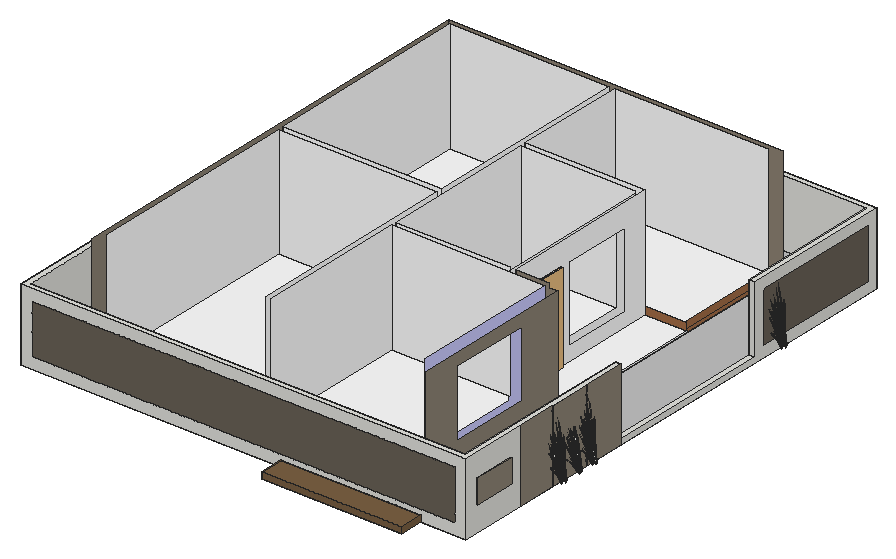
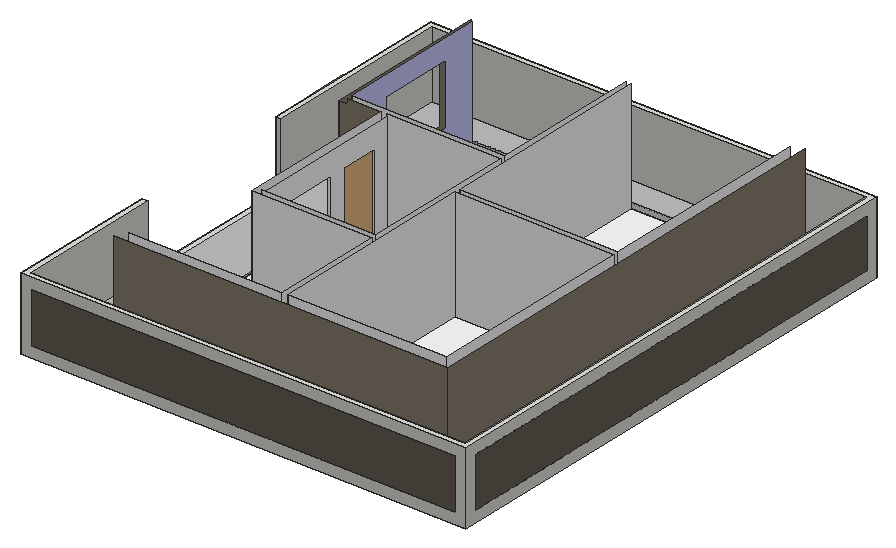
# SketchUp Ruby script. Lengths in inches.
U = 1.inch
M = Sketchup.active_model
def pt(a) = Geom::Point3d.new(a.map { |v| v * U })
def face(e, loops, mat)
  f = e.add_face(loops[0].map { |a| pt(a) })
  loops[1..].each { |l| e.add_face(l.map { |a| pt(a) }).erase! }
  f.material = f.back_material = mat if mat
  f
end
# faces: each face lists its corners as indices into pts; further lists are holes
def faces(e, pts, list, mat = nil) = list.each { |f| face(e, (f[0].is_a?(Array) ? f : [f]).map { |l| l.map { |i| pts[i] } }, mat) }
# xy, xz, yz: faces in a plane at the given z, y or x. An outline is a flat list of corners, or four numbers for a rectangle; further outlines are holes
def ring(l) = l.size == 4 ? [[l[0], l[1]], [l[2], l[1]], [l[2], l[3]], [l[0], l[3]]] : l.each_slice(2).to_a
def flat(e, list, mat, &to3) = list.each { |f| face(e, (f[0].is_a?(Array) ? f : [f]).map { |l| ring(l).map { |u, v| to3.(u, v) } }, mat) }
def xy(e, z, list, mat = nil) = flat(e, list, mat) { |x, y| [x, y, z] }
def xz(e, y, list, mat = nil) = flat(e, list, mat) { |x, z| [x, y, z] }
def yz(e, x, list, mat = nil) = flat(e, list, mat) { |y, z| [x, y, z] }
def lines(e, pts, list) = list.each { |a, b| e.add_line(pt(pts[a]), pt(pts[b])) }
# prism: a flat outline (further loops are holes) pulled along v
def prism(e, loops, v, mat = nil)
  f = face(e, loops, mat); d = Geom::Vector3d.new(v.map { |x| x * U })
  f.pushpull(f.normal.samedirection?(d) ? d.length : -d.length)
end
def box(e, o, s, mat = nil) = prism(e, [[o, [o[0] + s[0], o[1], o[2]], [o[0] + s[0], o[1] + s[1], o[2]], [o[0], o[1] + s[1], o[2]]]], [0, 0, s[2]], mat)
def at(x, y, z, deg = 0) = Geom::Transformation.translation(pt([x, y, z])) * Geom::Transformation.rotation(ORIGIN, Z_AXIS, deg.degrees)
def axes(o, x, y, z) = Geom::Transformation.new([*x, 0, *y, 0, *z, 0, *pt(o).to_a, 1])
def part(name) = M.definitions.add(name)
# library, detail: a bought-in or finely detailed component or shape, given as its bounding box
def library(name, o, s) = part(name).tap { |d| box(d.entities, o, s) }
def detail(e, o, s) = box(e.add_group.entities, o, s)
def put(e, d, t, mat = nil) = e.add_instance(d, t).tap { |i| i.material = mat if mat }
def group(e, t, mat = nil) = e.add_group.tap { |g| g.transformation = t; g.material = mat if mat }.entities
root = M.entities
M.materials.add("I01_Sky_Frost").color = [204, 204, 255]
M.materials.add("LightPink_Translucent").color = [144, 107, 117]
M.materials["LightPink_Translucent"].alpha = 0.75
M.materials.add("M00_Soft_Cloud").color = [255, 255, 255]
M.materials.add("M07_Charcoal_Gleam").color = [58, 58, 58]
M.materials.add("Plaster_04_1K").color = [142, 132, 117]
M.materials.add("Plaster_04_1K1").color = [106, 98, 87]
M.materials.add("Soil_03_1K").color = [122, 96, 67]
M.materials.add("Wood_Veneer_15_1K").color = [163, 109, 71]
M.materials.add("[Metal_Corrogated_Shiny]").color = [193, 193, 193]
c1 = library("porta+4",[0.2,-5.42,1.33],[46.55,4.72,83.21])
c2 = part("blade")
p = [[2.15,0.21,22],[0,0.17,0],[0.09,0.45,0],[2.18,0.31,22],[2.29,0.31,22],[0.38,0.45,0],
  [2.48,0.24,33],[2.49,0.24,33],[2.48,0.22,33]]
faces(c2.entities,p,[[0,1,2,3],[4,5,2,3],[6,3,4,7],[8,0,3,6]])
c3 = part("seeds")
p = [[0.3,-0.1,1.38],[-0.01,-0.03,1.59],[-0.01,-0.03,0.03],[0.14,-0.07,-0.07],[0.29,-0.03,3],[0.15,0.01,3.11]]
faces(c3.entities,p,[[0,1,2,3],[1,0,4,5]],"LightPink_Translucent")
c4 = part("blade with seeds")
put(c4.entities,c2,at(0,0,0))
put(c4.entities,c3,axes([2.4,0.25,30.99],[1.5799,-0.05474,1.17369],[-0.12525,1.92788,0.29478],[-0.07173,-0.02425,1.56792]))
xy(root,-6,[[280.62,2.62,431.17,27.98],[[0,27.98,480,579.98],[48.29,63.98,409.55,544.6]]])
xy(root,-6,[[48,63.98,408,543.98]],"M00_Soft_Cloud")
xy(root,0,[[474,236.51,480,416.03]])
xy(root,0,[[57,72.98,228,303.98],[234,72.98,399,234.98],[234,240.98,357,408.98],[363,240.98,408,414.98],[57,309.98,228,534.98],
  [234,414.98,399,534.98]],"M00_Soft_Cloud")
xy(root,0,[[[6,33.98,474,573.98],[48.29,63.98,409.55,544.6]]],"[Metal_Corrogated_Shiny]")
xy(root,0.58,[[280.62,2.62,431.17,27.98]],"Soil_03_1K")
xy(root,3,[[357,255.98,363,297.98]],"M00_Soft_Cloud")
xy(root,22.44,[[480,40.97,482,86.92]],"Plaster_04_1K")
xy(root,48.1875,[[480,40.97,482,86.92]],"Plaster_04_1K")
xy(root,72,[[0,27.98,480,27.98,480,236.51,474,236.51,474,33.98,6,33.98,6,573.98,474,573.98,474,416.03,480,416.03,480,579.98,0,579.98]])
xz(root,2.62,[[280.62,-6,431.17,0.58]],"Soil_03_1K")
xz(root,27.98,[[[0,-6,280.62,-6,280.62,0.58,431.17,0.58,431.17,-6,480,-6,480,72,0,72],[12,6,468,60]],[280.62,-6,431.17,0.58]])
xz(root,27.98,[[12,6,468,60]],"Plaster_04_1K1")
xz(root,33.98,[[6,0,474,72]])
xz(root,40.97,[[480,22.44,482,48.1875]],"Plaster_04_1K")
xz(root,63.98,[[48,-6,48.29,0],[48.29,-6,409.55,0]])
xz(root,86.92,[[480,22.44,482,48.1875]],"Plaster_04_1K")
xz(root,234.98,[[234,0,399,120]],"M00_Soft_Cloud")
xz(root,236.51,[[474,0,480,72]])
xz(root,240.98,[[234,0,357,120]],"M00_Soft_Cloud")
xz(root,240.98,[[363,0,363,120,399,120,399,114.97,408,114.97,408,0]],"Plaster_04_1K")
xz(root,255.98,[[357,3,363,93]],"M00_Soft_Cloud")
xz(root,297.98,[[357,3,363,93]],"M00_Soft_Cloud")
xz(root,303.98,[[57,0,228,120]],"M00_Soft_Cloud")
xz(root,309.98,[[57,0,228,120]],"M00_Soft_Cloud")
xz(root,408.98,[[234,0,357,120]],"M00_Soft_Cloud")
xz(root,414.98,[[234,0,363,120]],"M00_Soft_Cloud")
xz(root,414.98,[[363,0,408,8.21]],"Wood_Veneer_15_1K")
xz(root,416.03,[[474,0,480,72]])
xz(root,534.98,[[57,0,228,120],[234,0,399,120]],"M00_Soft_Cloud")
xz(root,543.98,[[48,-6,408,117]],"Plaster_04_1K")
xz(root,544.6,[[48.29,-6,409.55,0]])
xz(root,573.98,[[6,0,474,72]])
xz(root,579.98,[[[0,-6,480,72],[12,6,468,60]]])
xz(root,579.98,[[12,6,468,60]],"Plaster_04_1K1")
yz(root,0,[[[27.98,-6,579.98,72],[39.98,6,567.98,60]]])
yz(root,0,[[39.98,6,567.98,60]],"Plaster_04_1K1")
yz(root,6,[[33.98,0,573.98,72]])
yz(root,48,[[63.98,-6,543.98,117]],"Plaster_04_1K")
yz(root,48.29,[[63.98,-6,544.6,0]])
yz(root,57,[[72.98,0,303.98,120],[309.98,0,534.98,120]],"M00_Soft_Cloud")
yz(root,228,[[72.98,0,303.98,120],[309.98,0,534.98,120]],"M00_Soft_Cloud")
yz(root,234,[[72.98,0,234.98,120],[240.98,0,408.98,120],[414.98,0,534.98,120]],"M00_Soft_Cloud")
yz(root,280.62,[[2.62,-6,27.98,0.58]],"Soil_03_1K")
yz(root,357,[[[240.98,0,408.98,117],[315.98,18,384.98,93],[255.98,3,297.98,93]]],"M00_Soft_Cloud")
yz(root,363,[[[240.98,0,252.98,0,252.98,96,300.98,96,300.98,0,414.98,0,414.98,120,240.98,120],[312.98,15,387.98,96]],[[252.98,0,300.98,96],[255.98,3,297.98,93]]],"M00_Soft_Cloud")
yz(root,399,[[[72.98,0,234.98,120],[111.98,30,186.98,30,186.98,33,189.98,33,189.98,99,108.98,99,108.98,33,111.98,33]]],"I01_Sky_Frost")
yz(root,408,[[240.98,-6,414.98,0]],"M00_Soft_Cloud")
yz(root,408,[[[63.98,-6,240.98,114.97],[105.98,30,192.98,102]]],"Plaster_04_1K")
yz(root,408,[[414.98,-6,543.98,2.03],[414.98,2.03,543.98,10.05]],"Wood_Veneer_15_1K")
yz(root,409.55,[[63.98,-6,544.6,0]])
yz(root,431.17,[[2.62,-6,27.98,0.58]],"Soil_03_1K")
yz(root,474,[[33.98,0,236.51,72],[416.03,0,573.98,72]])
yz(root,480,[[[27.98,-6,99.98,72],[40.97,22.44,86.92,48.1875]],[[236.51,-6,579.98,-6,579.98,72,416.03,72,416.03,0,236.51,0],[428.03,6,567.98,60]]])
yz(root,480,[[143.49,-6,145.49,72],[189,-6,191,72]],"M07_Charcoal_Gleam")
yz(root,480,[[99.98,-6,143.49,72],[145.49,-6,189,72],[191,-6,236.51,72]],"Plaster_04_1K")
yz(root,480,[[428.03,6,567.98,60]],"Plaster_04_1K1")
yz(root,482,[[40.97,22.44,86.92,48.1875]],"Plaster_04_1K")
p = [[363,408.98,0],[357,408.98,0]]
lines(root,p,[[0,1]])
put(root,c1,axes([360.24,254.23,-1.54],[0,1,0],[-1,0,0],[0,0,1.15408]))
put(root,c4,axes([489.51,442.16,3.07],[0.31515,-0.01384,1.71376],[-0.20907,0.5998,0.13857],[-0.44912,-0.0371,0.73262]))
put(root,c4,axes([489.58,145.76,3.07],[0.31515,-0.01384,1.71376],[-0.20907,0.5998,0.13857],[-0.44912,-0.0371,0.73262]))
put(root,c4,axes([489.65,186.83,3.07],[0.31515,-0.01384,1.71376],[-0.20907,0.5998,0.13857],[-0.44912,-0.0371,0.73262]))
put(root,c4,axes([489.64,443.21,3.07],[0.26363,-0.12925,1.71376],[0.22195,0.59723,0.13857],[-0.41388,0.13498,0.73262]))
put(root,c4,axes([489.71,146.8125,3.07],[0.26363,-0.12925,1.71376],[0.22195,0.59723,0.13857],[-0.41388,0.13498,0.73262]))
put(root,c4,axes([489.78,187.88,3.07],[0.26363,-0.12925,1.71376],[0.22195,0.59723,0.13857],[-0.41388,0.13498,0.73262]))
put(root,c4,axes([488.82,444.23,1.78],[0.26405,0.05016,1.43002],[0.17019,0.51235,-0.30754],[-0.35868,0.0959,0.61141]))
put(root,c4,axes([488.89,147.83,1.78],[0.26405,0.05016,1.43002],[0.17019,0.51235,-0.30754],[-0.35868,0.0959,0.61141]))
put(root,c4,axes([488.96,188.9,1.78],[0.26405,0.05016,1.43002],[0.17019,0.51235,-0.30754],[-0.35868,0.0959,0.61141]))
put(root,c4,axes([491.15,442.59,2.53],[0.21597,-0.08839,1.77064],[0.07448,0.61717,0.13857],[-0.4678,0.08189,0.63284]))
put(root,c4,axes([491.23,146.1875,2.53],[0.21597,-0.08839,1.77064],[0.07448,0.61717,0.13857],[-0.4678,0.08189,0.63284]))
put(root,c4,axes([491.3,187.26,2.53],[0.21597,-0.08839,1.77064],[0.07448,0.61717,0.13857],[-0.4678,0.08189,0.63284]))
put(root,c4,axes([491.2,165.89,3.07],[0.31515,-0.01384,1.71376],[-0.20907,0.5998,0.13857],[-0.44912,-0.0371,0.73262]))
put(root,c4,axes([488.83,443,3.91],[-0.12407,0.07933,1.74944],[0.01055,0.57963,-0.27667],[-0.2844,0.07538,0.14031]))
put(root,c4,axes([490.45,441.6,4.17],[-0.75952,-0.01471,-0.71045],[0.05101,-0.61953,0.08574],[-0.32177,-0.06538,1.00501]))
put(root,c4,axes([488.91,146.6,3.91],[-0.12407,0.07933,1.74944],[0.01055,0.57963,-0.27667],[-0.2844,0.07538,0.14031]))
put(root,c4,axes([490.53,145.2,4.17],[-0.75952,-0.01471,-0.71045],[0.05101,-0.61953,0.08574],[-0.32177,-0.06538,1.00501]))
put(root,c4,axes([489.84,441.75,1.78],[0.14835,0.17012,1.43002],[-0.34183,0.46242,-0.30754],[-0.351,-0.11053,0.61141]))
put(root,c4,axes([488.98,187.67,3.91],[-0.12407,0.07933,1.74944],[0.01055,0.57963,-0.27667],[-0.2844,0.07538,0.14031]))
put(root,c4,axes([490.59,186.27,4.17],[-0.75952,-0.01471,-0.71045],[0.05101,-0.61953,0.08574],[-0.32177,-0.06538,1.00501]))
put(root,c4,axes([489.91,145.35,1.78],[0.14835,0.17012,1.43002],[-0.34183,0.46242,-0.30754],[-0.351,-0.11053,0.61141]))
put(root,c4,axes([489.23,442.67,3.72],[-0.63144,-0.17046,-0.35414],[0.18417,-0.49731,0.4572],[-0.25423,0.0456,0.87481]))
put(root,c4,axes([489.98,186.42,1.78],[0.14835,0.17012,1.43002],[-0.34183,0.46242,-0.30754],[-0.351,-0.11053,0.61141]))
put(root,c4,axes([490.1,441.19,3.07],[0.28223,0.10528,1.71376],[-0.58406,0.44165,0.13857],[-0.36402,-0.19924,0.73262]))
put(root,c4,axes([489.3,146.27,3.72],[-0.63144,-0.17046,-0.35414],[0.18417,-0.49731,0.4572],[-0.25423,0.0456,0.87481]))
put(root,c4,axes([490.18,144.79,3.07],[0.28223,0.10528,1.71376],[-0.58406,0.44165,0.13857],[-0.36402,-0.19924,0.73262]))
put(root,c4,axes([489.375,187.34,3.72],[-0.63144,-0.17046,-0.35414],[0.18417,-0.49731,0.4572],[-0.25423,0.0456,0.87481]))
put(root,c4,axes([490.25,185.86,3.07],[0.28223,0.10528,1.71376],[-0.58406,0.44165,0.13857],[-0.36402,-0.19924,0.73262]))
put(root,c4,axes([487.45,443.59,3.9],[0.09697,0.01639,1.77383],[0.29997,0.53988,-0.16761],[-0.1985,0.1417,0.31391]))
put(root,c4,axes([489.66,442.92,3.875],[-0.20584,0.55581,-0.51099],[-0.70573,-0.19051,-0.3958],[-0.28414,0.05097,0.97773]))
put(root,c4,axes([487.53,147.1875,3.9],[0.09697,0.01639,1.77383],[0.29997,0.53988,-0.16761],[-0.1985,0.1417,0.31391]))
put(root,c4,axes([489.74,146.53,3.875],[-0.20584,0.55581,-0.51099],[-0.70573,-0.19051,-0.3958],[-0.28414,0.05097,0.97773]))
put(root,c4,axes([487.6,188.26,3.9],[0.09697,0.01639,1.77383],[0.29997,0.53988,-0.16761],[-0.1985,0.1417,0.31391]))
put(root,c4,axes([489.81,187.59,3.875],[-0.20584,0.55581,-0.51099],[-0.70573,-0.19051,-0.3958],[-0.28414,0.05097,0.97773]))
put(root,c4,axes([490.2,441.72,3.875],[-0.55171,0.40476,-0.51099],[-0.48318,-0.42758,-0.3958],[-0.28031,-0.06159,0.97773]))
put(root,c4,axes([489.31,442.89,0.6875],[0.01927,0.0963,1.76342],[-0.38846,0.5029,-0.26939],[-0.27592,-0.02535,0.30037]))
put(root,c4,axes([491.33,166.95,3.07],[0.26363,-0.12925,1.71376],[0.22195,0.59723,0.13857],[-0.41388,0.13498,0.73262]))
put(root,c4,axes([490.27,145.32,3.875],[-0.55171,0.40476,-0.51099],[-0.48318,-0.42758,-0.3958],[-0.28031,-0.06159,0.97773]))
put(root,c4,axes([489.38,146.49,0.6875],[0.01927,0.0963,1.76342],[-0.38846,0.5029,-0.26939],[-0.27592,-0.02535,0.30037]))
put(root,c4,axes([490.34,186.39,3.875],[-0.55171,0.40476,-0.51099],[-0.48318,-0.42758,-0.3958],[-0.28031,-0.06159,0.97773]))
put(root,c4,axes([489.45,187.56,0.6875],[0.01927,0.0963,1.76342],[-0.38846,0.5029,-0.26939],[-0.27592,-0.02535,0.30037]))
put(root,c4,axes([490.51,167.97,1.78],[0.26405,0.05016,1.43002],[0.17019,0.51235,-0.30754],[-0.35868,0.0959,0.61141]))
put(root,c4,axes([489.42,440.59,3.9],[0.05633,0.06098,1.77383],[-0.27155,0.54815,-0.16761],[-0.27501,0.00397,0.31391]))
put(root,c4,axes([489.49,144.19,3.9],[0.05633,0.06098,1.77383],[-0.27155,0.54815,-0.16761],[-0.27501,0.00397,0.31391]))
put(root,c4,axes([488.26,445.3,1.96],[0.31665,-0.27694,1.1486],[0.12495,0.43841,0.84392],[-0.22883,0.0785,0.25299]))
put(root,c4,axes([489.5625,185.26,3.9],[0.05633,0.06098,1.77383],[-0.27155,0.54815,-0.16761],[-0.27501,0.00397,0.31391]))
put(root,c4,axes([490.05,440.22,3.91],[-0.16348,-0.00431,1.74944],[-0.52047,0.43131,-0.27667],[-0.2777,-0.08813,0.14031]))
put(root,c4,axes([488.34,148.9,1.96],[0.31665,-0.27694,1.1486],[0.12495,0.43841,0.84392],[-0.22883,0.0785,0.25299]))
put(root,c4,axes([492.85,166.33,2.53],[0.21597,-0.08839,1.77064],[0.07448,0.61717,0.13857],[-0.4678,0.08189,0.63284]))
put(root,c4,axes([488.41,189.97,1.96],[0.31665,-0.27694,1.1486],[0.12495,0.43841,0.84392],[-0.22883,0.0785,0.25299]))
put(root,c4,axes([490.12,143.82,3.91],[-0.16348,-0.00431,1.74944],[-0.52047,0.43131,-0.27667],[-0.2777,-0.08813,0.14031]))
put(root,c4,axes([489.375,442.61,3.93],[0.21466,-0.55714,0.48003],[0.70573,0.19051,0.3958],[-0.27753,0.03348,0.9933]))
put(root,c4,axes([490.19,184.89,3.91],[-0.16348,-0.00431,1.74944],[-0.52047,0.43131,-0.27667],[-0.2777,-0.08813,0.14031]))
put(root,c4,axes([489.625,442.45,4.23],[0.38229,0.5533,-0.1216],[-0.6785,0.2719,-0.67495],[-0.28593,0.073,1.02557]))
put(root,c4,axes([489.45,146.21,3.93],[0.21466,-0.55714,0.48003],[0.70573,0.19051,0.3958],[-0.27753,0.03348,0.9933]))
put(root,c4,axes([490.49,441.3,4.23],[-0.04068,0.62141,-0.1216],[-0.77029,-0.01698,-0.67495],[-0.29667,-0.04317,1.02557]))
put(root,c4,axes([489.99,441.34,3.72],[-0.43232,-0.38257,-0.35414],[0.49364,-0.36215,0.4572],[-0.25081,-0.0551,0.87481]))
put(root,c4,axes([489.7,146.05,4.23],[0.38229,0.5533,-0.1216],[-0.6785,0.2719,-0.67495],[-0.28593,0.073,1.02557]))
put(root,c4,axes([489.52,187.28,3.93],[0.21466,-0.55714,0.48003],[0.70573,0.19051,0.3958],[-0.27753,0.03348,0.9933]))
put(root,c4,axes([489.32,442.46,3.92],[-0.27906,-0.41663,0.0643],[0.50888,-0.20393,0.50621],[-0.22432,0.04024,0.77189]))
put(root,c4,axes([490.5625,144.9,4.23],[-0.04068,0.62141,-0.1216],[-0.77029,-0.01698,-0.67495],[-0.29667,-0.04317,1.02557]))
put(root,c4,axes([490.07,144.94,3.72],[-0.43232,-0.38257,-0.35414],[0.49364,-0.36215,0.4572],[-0.25081,-0.0551,0.87481]))
put(root,c4,axes([489.77,187.12,4.23],[0.38229,0.5533,-0.1216],[-0.6785,0.2719,-0.67495],[-0.28593,0.073,1.02557]))
put(root,c4,axes([490.6,443.61,3.07],[0.18977,-0.18775,1.71376],[0.47917,0.50677,0.13857],[-0.32866,0.23079,0.73262]))
put(root,c4,axes([489.46,444.11,3.72],[-0.66138,0.08733,-0.35414],[-0.17464,-0.49921,0.4572],[-0.18953,0.13408,0.87481]))
put(root,c4,axes([489.4,146.0625,3.92],[-0.27906,-0.41663,0.0643],[0.50888,-0.20393,0.50621],[-0.22432,0.04024,0.77189]))
put(root,c4,axes([490.63,185.97,4.23],[-0.04068,0.62141,-0.1216],[-0.77029,-0.01698,-0.67495],[-0.29667,-0.04317,1.02557]))
put(root,c4,axes([490.14,186.01,3.72],[-0.43232,-0.38257,-0.35414],[0.49364,-0.36215,0.4572],[-0.25081,-0.0551,0.87481]))
put(root,c4,axes([490.68,147.21,3.07],[0.18977,-0.18775,1.71376],[0.47917,0.50677,0.13857],[-0.32866,0.23079,0.73262]))
put(root,c4,axes([489.47,187.13,3.92],[-0.27906,-0.41663,0.0643],[0.50888,-0.20393,0.50621],[-0.22432,0.04024,0.77189]))
put(root,c4,axes([489.54,147.71,3.72],[-0.66138,0.08733,-0.35414],[-0.17464,-0.49921,0.4572],[-0.18953,0.13408,0.87481]))
put(root,c4,axes([490.75,188.28,3.07],[0.18977,-0.18775,1.71376],[0.47917,0.50677,0.13857],[-0.32866,0.23079,0.73262]))
put(root,c4,axes([489.61,188.78,3.72],[-0.66138,0.08733,-0.35414],[-0.17464,-0.49921,0.4572],[-0.18953,0.13408,0.87481]))
put(root,c4,axes([489.1,445.59,0.6875],[0.10192,0.06105,1.76342],[0.17281,0.56562,-0.26939],[-0.22588,0.12062,0.30037]))
put(root,c4,axes([490.53,166.74,3.91],[-0.12407,0.07933,1.74944],[0.01055,0.57963,-0.27667],[-0.2844,0.07538,0.14031]))
put(root,c4,axes([492.14,165.34,4.17],[-0.75952,-0.01471,-0.71045],[0.05101,-0.61953,0.08574],[-0.32177,-0.06538,1.00501]))
put(root,c4,axes([488.95,442.26,1.96],[0.48508,-0.04372,1.1486],[-0.3077,0.38525,0.84392],[-0.23971,-0.05779,0.25299]))
put(root,c4,axes([489.18,149.1875,0.6875],[0.10192,0.06105,1.76342],[0.17281,0.56562,-0.26939],[-0.22588,0.12062,0.30037]))
put(root,c4,axes([491.53,165.49,1.78],[0.14835,0.17012,1.43002],[-0.34183,0.46242,-0.30754],[-0.351,-0.11053,0.61141]))
put(root,c4,axes([489.03,145.86,1.96],[0.48508,-0.04372,1.1486],[-0.3077,0.38525,0.84392],[-0.23971,-0.05779,0.25299]))
put(root,c4,axes([489.24,190.26,0.6875],[0.10192,0.06105,1.76342],[0.17281,0.56562,-0.26939],[-0.22588,0.12062,0.30037]))
put(root,c4,axes([489.1,186.93,1.96],[0.48508,-0.04372,1.1486],[-0.3077,0.38525,0.84392],[-0.23971,-0.05779,0.25299]))
put(root,c4,axes([490.92,166.41,3.72],[-0.63144,-0.17046,-0.35414],[0.18417,-0.49731,0.4572],[-0.25423,0.0456,0.87481]))
put(root,c4,axes([489.54,444,3.93],[-0.18844,-0.56237,0.48003],[0.73919,-0.0976,0.3958],[-0.21785,0.13226,0.9933]))
put(root,c4,axes([491.8,164.93,3.07],[0.28223,0.10528,1.71376],[-0.58406,0.44165,0.13857],[-0.36402,-0.19924,0.73262]))
put(root,c4,axes([489.62,147.6,3.93],[-0.18844,-0.56237,0.48003],[0.73919,-0.0976,0.3958],[-0.21785,0.13226,0.9933]))
put(root,c4,axes([489.93,441.2,4.29],[0.62747,-0.45094,0.53763],[0.54116,0.47889,0.4433],[-0.29439,-0.08318,1.11249]))
put(root,c4,axes([489.69,188.67,3.93],[-0.18844,-0.56237,0.48003],[0.73919,-0.0976,0.3958],[-0.21785,0.13226,0.9933]))
put(root,c4,axes([489.4,443.89,3.92],[-0.52161,-0.25698,0.0643],[0.30368,-0.36595,0.50621],[-0.16723,0.11831,0.77189]))
put(root,c4,axes([490,144.8,4.29],[0.62747,-0.45094,0.53763],[0.54116,0.47889,0.4433],[-0.29439,-0.08318,1.11249]))
put(root,c4,axes([489.15,167.33,3.9],[0.09697,0.01639,1.77383],[0.29997,0.53988,-0.16761],[-0.1985,0.1417,0.31391]))
put(root,c4,axes([489.48,147.49,3.92],[-0.52161,-0.25698,0.0643],[0.30368,-0.36595,0.50621],[-0.16723,0.11831,0.77189]))
put(root,c4,axes([490.07,185.87,4.29],[0.62747,-0.45094,0.53763],[0.54116,0.47889,0.4433],[-0.29439,-0.08318,1.11249]))
put(root,c4,axes([491.36,166.66,3.875],[-0.20584,0.55581,-0.51099],[-0.70573,-0.19051,-0.3958],[-0.28414,0.05097,0.97773]))
put(root,c4,axes([489.55,188.56,3.92],[-0.52161,-0.25698,0.0643],[0.30368,-0.36595,0.50621],[-0.16723,0.11831,0.77189]))
put(root,c4,axes([491.89,165.46,3.875],[-0.55171,0.40476,-0.51099],[-0.48318,-0.42758,-0.3958],[-0.28031,-0.06159,0.97773]))
put(root,c4,axes([490.46,444.08,3.07],[0.14147,-0.21002,1.71376],[0.59349,0.43464,0.13857],[-0.26773,0.27089,0.73262]))
put(root,c4,axes([491,166.63,0.6875],[0.01927,0.0963,1.76342],[-0.38846,0.5029,-0.26939],[-0.27592,-0.02535,0.30037]))
put(root,c4,axes([490.54,147.68,3.07],[0.14147,-0.21002,1.71376],[0.59349,0.43464,0.13857],[-0.26773,0.27089,0.73262]))
put(root,c4,axes([490.61,188.75,3.07],[0.14147,-0.21002,1.71376],[0.59349,0.43464,0.13857],[-0.26773,0.27089,0.73262]))
put(root,c4,axes([491.11,164.33,3.9],[0.05633,0.06098,1.77383],[-0.27155,0.54815,-0.16761],[-0.27501,0.00397,0.31391]))
put(root,c4,axes([489.89,442.62,4.24],[0.63144,0.17046,0.35414],[-0.18417,0.49731,-0.4572],[-0.25423,0.0456,0.87481]))
put(root,c4,axes([489.97,146.22,4.24],[0.63144,0.17046,0.35414],[-0.18417,0.49731,-0.4572],[-0.25423,0.0456,0.87481]))
put(root,c4,axes([490,444.16,3.875],[0.19519,0.55794,-0.51099],[-0.73919,0.0976,-0.3958],[-0.21183,0.14986,0.97773]))
put(root,c4,axes([489.96,169.04,1.96],[0.31665,-0.27694,1.1486],[0.12495,0.43841,0.84392],[-0.22883,0.0785,0.25299]))
put(root,c4,axes([490.04,187.29,4.24],[0.63144,0.17046,0.35414],[-0.18417,0.49731,-0.4572],[-0.25423,0.0456,0.87481]))
put(root,c4,axes([491.74,163.96,3.91],[-0.16348,-0.00431,1.74944],[-0.52047,0.43131,-0.27667],[-0.2777,-0.08813,0.14031]))
put(root,c4,axes([490.08,147.76,3.875],[0.19519,0.55794,-0.51099],[-0.73919,0.0976,-0.3958],[-0.21183,0.14986,0.97773]))
put(root,c4,axes([490.21,441.2,3.92],[0.03826,-0.46465,0.0643],[0.57772,0.01274,0.50621],[-0.2213,-0.04862,0.77189]))
put(root,c4,axes([488.85,445.17,3.91],[-0.01889,0.12092,1.74944],[0.53598,0.42065,-0.27667],[-0.14032,0.19892,0.14031]))
put(root,c4,axes([490.15,188.83,3.875],[0.19519,0.55794,-0.51099],[-0.73919,0.0976,-0.3958],[-0.21183,0.14986,0.97773]))
put(root,c4,axes([490.29,144.8,3.92],[0.03826,-0.46465,0.0643],[0.57772,0.01274,0.50621],[-0.2213,-0.04862,0.77189]))
put(root,c4,axes([488.93,148.77,3.91],[-0.01889,0.12092,1.74944],[0.53598,0.42065,-0.27667],[-0.14032,0.19892,0.14031]))
put(root,c4,axes([491.85,443.76,1.25],[-0.79037,-0.10018,-0.62353],[0.16679,-0.61794,-0.16365],[-0.23587,-0.07488,1.37633]))
put(root,c4,axes([491.99,440.39,4.62],[-0.50709,0.58578,-0.13619],[-0.73436,-0.33748,-0.75594],[-0.25527,-0.1655,1.14864]))
put(root,c4,axes([491.07,166.35,3.93],[0.21466,-0.55714,0.48003],[0.70573,0.19051,0.3958],[-0.27753,0.03348,0.9933]))
put(root,c4,axes([490.36,185.87,3.92],[0.03826,-0.46465,0.0643],[0.57772,0.01274,0.50621],[-0.2213,-0.04862,0.77189]))
put(root,c4,axes([489,189.84,3.91],[-0.01889,0.12092,1.74944],[0.53598,0.42065,-0.27667],[-0.14032,0.19892,0.14031]))
put(root,c4,axes([491.92,147.36,1.25],[-0.79037,-0.10018,-0.62353],[0.16679,-0.61794,-0.16365],[-0.23587,-0.07488,1.37633]))
put(root,c4,axes([491.32,166.1875,4.23],[0.38229,0.5533,-0.1216],[-0.6785,0.2719,-0.67495],[-0.28593,0.073,1.02557]))
put(root,c4,axes([492.07,143.99,4.62],[-0.50709,0.58578,-0.13619],[-0.73436,-0.33748,-0.75594],[-0.25527,-0.1655,1.14864]))
put(root,c4,axes([490.6,441.54,4.24],[0.43232,0.38257,0.35414],[-0.49364,0.36215,-0.4572],[-0.25081,-0.0551,0.87481]))
put(root,c4,axes([492.18,165.04,4.23],[-0.04068,0.62141,-0.1216],[-0.77029,-0.01698,-0.67495],[-0.29667,-0.04317,1.02557]))
put(root,c4,axes([491.99,188.43,1.25],[-0.79037,-0.10018,-0.62353],[0.16679,-0.61794,-0.16365],[-0.23587,-0.07488,1.37633]))
put(root,c4,axes([491.6875,165.08,3.72],[-0.43232,-0.38257,-0.35414],[0.49364,-0.36215,0.4572],[-0.25081,-0.0551,0.87481]))
put(root,c4,axes([492.14,185.0625,4.62],[-0.50709,0.58578,-0.13619],[-0.73436,-0.33748,-0.75594],[-0.25527,-0.1655,1.14864]))
put(root,c4,axes([491.02,166.2,3.92],[-0.27906,-0.41663,0.0643],[0.50888,-0.20393,0.50621],[-0.22432,0.04024,0.77189]))
put(root,c4,axes([490.68,145.14,4.24],[0.43232,0.38257,0.35414],[-0.49364,0.36215,-0.4572],[-0.25081,-0.0551,0.87481]))
put(root,c4,axes([491.77,440.87,4.17],[-0.64788,-0.29534,-0.71045],[0.46044,-0.51755,0.08574],[-0.23473,-0.17635,1.00501]))
put(root,c4,axes([491.47,440.88,3.875],[-0.74975,0.14525,-0.51099],[-0.13115,-0.55007,-0.3958],[-0.20138,-0.15763,0.97773]))
put(root,c4,axes([492.3,167.35,3.07],[0.18977,-0.18775,1.71376],[0.47917,0.50677,0.13857],[-0.32866,0.23079,0.73262]))
put(root,c4,axes([490.75,186.21,4.24],[0.43232,0.38257,0.35414],[-0.49364,0.36215,-0.4572],[-0.25081,-0.0551,0.87481]))
put(root,c4,axes([491.16,167.84,3.72],[-0.66138,0.08733,-0.35414],[-0.17464,-0.49921,0.4572],[-0.18953,0.13408,0.87481]))
put(root,c4,axes([491.85,144.47,4.17],[-0.64788,-0.29534,-0.71045],[0.46044,-0.51755,0.08574],[-0.23473,-0.17635,1.00501]))
put(root,c4,axes([491.54,144.48,3.875],[-0.74975,0.14525,-0.51099],[-0.13115,-0.55007,-0.3958],[-0.20138,-0.15763,0.97773]))
put(root,c4,axes([491.91,185.54,4.17],[-0.64788,-0.29534,-0.71045],[0.46044,-0.51755,0.08574],[-0.23473,-0.17635,1.00501]))
put(root,c4,axes([491.61,185.55,3.875],[-0.74975,0.14525,-0.51099],[-0.13115,-0.55007,-0.3958],[-0.20138,-0.15763,0.97773]))
put(root,c4,axes([490.8,169.33,0.6875],[0.10192,0.06105,1.76342],[0.17281,0.56562,-0.26939],[-0.22588,0.12062,0.30037]))
put(root,c4,axes([490.81,444.93,1.21],[-0.7111,-0.30552,-0.49651],[0.42504,-0.54784,0],[-0.16196,-0.06958,1.57504]))
put(root,c4,axes([490.65,166,1.96],[0.48508,-0.04372,1.1486],[-0.3077,0.38525,0.84392],[-0.23971,-0.05779,0.25299]))
put(root,c4,axes([490.5,440.38,0.6875],[-0.0736,0.08049,1.76342],[-0.74378,0.17355,-0.26939],[-0.17968,-0.15788,0.30037]))
put(root,c4,axes([489.66,443.76,4.23],[0.70283,0.33692,-0.1216],[-0.40491,0.48793,-0.67495],[-0.19857,0.16961,1.02557]))
put(root,c4,axes([490.89,148.53,1.21],[-0.7111,-0.30552,-0.49651],[0.42504,-0.54784,0],[-0.16196,-0.06958,1.57504]))
put(root,c4,axes([490.58,143.98,0.6875],[-0.0736,0.08049,1.76342],[-0.74378,0.17355,-0.26939],[-0.17968,-0.15788,0.30037]))
put(root,c4,axes([489.73,147.36,4.23],[0.70283,0.33692,-0.1216],[-0.40491,0.48793,-0.67495],[-0.19857,0.16961,1.02557]))
put(root,c4,axes([490.96,189.6,1.21],[-0.7111,-0.30552,-0.49651],[0.42504,-0.54784,0],[-0.16196,-0.06958,1.57504]))
put(root,c4,axes([491.24,445.3,1.57],[-0.47504,0.61229,0],[-0.79476,-0.34146,-0.51607],[-0.18101,-0.07777,1.63711]))
put(root,c4,axes([490.64,185.05,0.6875],[-0.0736,0.08049,1.76342],[-0.74378,0.17355,-0.26939],[-0.17968,-0.15788,0.30037]))
put(root,c4,axes([489.8,188.43,4.23],[0.70283,0.33692,-0.1216],[-0.40491,0.48793,-0.67495],[-0.19857,0.16961,1.02557]))
put(root,c4,axes([491.24,167.74,3.93],[-0.18844,-0.56237,0.48003],[0.73919,-0.0976,0.3958],[-0.21785,0.13226,0.9933]))
put(root,c4,axes([491.32,148.9,1.57],[-0.47504,0.61229,0],[-0.79476,-0.34146,-0.51607],[-0.18101,-0.07777,1.63711]))
put(root,c4,axes([491.39,189.97,1.57],[-0.47504,0.61229,0],[-0.79476,-0.34146,-0.51607],[-0.18101,-0.07777,1.63711]))
